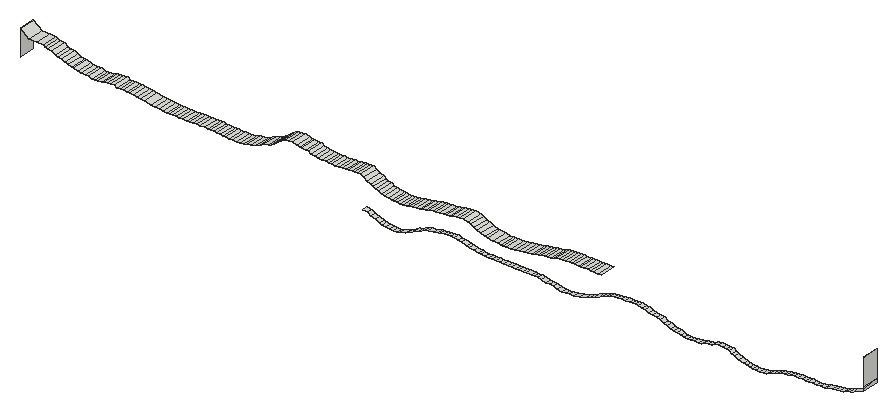
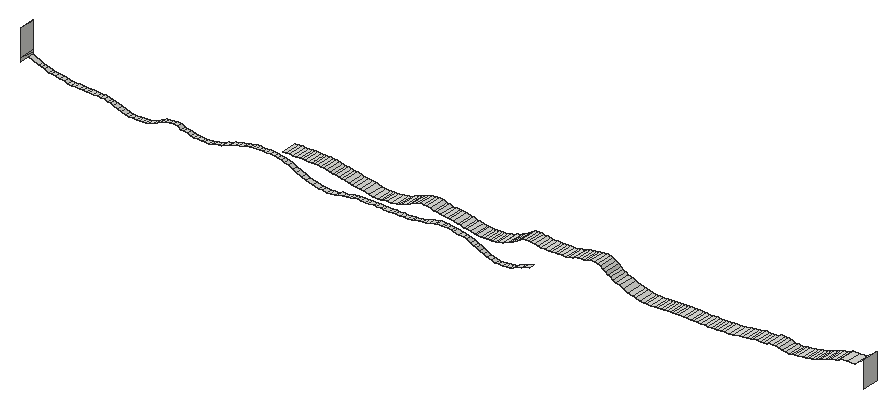
# SketchUp Ruby script. Lengths in inches.
U = 1.inch
M = Sketchup.active_model
def pt(a) = Geom::Point3d.new(a.map { |v| v * U })
def face(e, loops, mat)
  f = e.add_face(loops[0].map { |a| pt(a) })
  loops[1..].each { |l| e.add_face(l.map { |a| pt(a) }).erase! }
  f.material = f.back_material = mat if mat
  f
end
# faces: each face lists its corners as indices into pts; further lists are holes
def faces(e, pts, list, mat = nil) = list.each { |f| face(e, (f[0].is_a?(Array) ? f : [f]).map { |l| l.map { |i| pts[i] } }, mat) }
# xy, xz, yz: faces in a plane at the given z, y or x. An outline is a flat list of corners, or four numbers for a rectangle; further outlines are holes
def ring(l) = l.size == 4 ? [[l[0], l[1]], [l[2], l[1]], [l[2], l[3]], [l[0], l[3]]] : l.each_slice(2).to_a
def flat(e, list, mat, &to3) = list.each { |f| face(e, (f[0].is_a?(Array) ? f : [f]).map { |l| ring(l).map { |u, v| to3.(u, v) } }, mat) }
def xy(e, z, list, mat = nil) = flat(e, list, mat) { |x, y| [x, y, z] }
def xz(e, y, list, mat = nil) = flat(e, list, mat) { |x, z| [x, y, z] }
def yz(e, x, list, mat = nil) = flat(e, list, mat) { |y, z| [x, y, z] }
def lines(e, pts, list) = list.each { |a, b| e.add_line(pt(pts[a]), pt(pts[b])) }
# prism: a flat outline (further loops are holes) pulled along v
def prism(e, loops, v, mat = nil)
  f = face(e, loops, mat); d = Geom::Vector3d.new(v.map { |x| x * U })
  f.pushpull(f.normal.samedirection?(d) ? d.length : -d.length)
end
def box(e, o, s, mat = nil) = prism(e, [[o, [o[0] + s[0], o[1], o[2]], [o[0] + s[0], o[1] + s[1], o[2]], [o[0], o[1] + s[1], o[2]]]], [0, 0, s[2]], mat)
def at(x, y, z, deg = 0) = Geom::Transformation.translation(pt([x, y, z])) * Geom::Transformation.rotation(ORIGIN, Z_AXIS, deg.degrees)
def axes(o, x, y, z) = Geom::Transformation.new([*x, 0, *y, 0, *z, 0, *pt(o).to_a, 1])
def part(name) = M.definitions.add(name)
# library, detail: a bought-in or finely detailed component or shape, given as its bounding box
def library(name, o, s) = part(name).tap { |d| box(d.entities, o, s) }
def detail(e, o, s) = box(e.add_group.entities, o, s)
def put(e, d, t, mat = nil) = e.add_instance(d, t).tap { |i| i.material = mat if mat }
def group(e, t, mat = nil) = e.add_group.tap { |g| g.transformation = t; g.material = mat if mat }.entities
root = M.entities
xy(root,238.18,[[2133.53,2401.37,2134.21,2402.3]])
xy(root,238.62,[[2100.06,2401.37,2100.83,2402.3],[2100.83,2401.37,2101.46,2402.3],[2101.46,2401.37,2102.22,2402.3],[2102.22,2401.37,2102.84,2402.3],[2102.84,2401.37,2103.69,2402.3],
  [2103.69,2401.37,2104.33,2402.3],[2104.33,2401.37,2104.95,2402.3]])
xy(root,238.625,[[2098.64,2401.37,2099.5,2402.3]])
xy(root,238.89,[[2154.45,2401.37,2155.13,2402.3]])
xy(root,238.9,[[2155.89,2401.37,2156.51,2402.3],[2156.51,2401.37,2157.28,2402.3]])
xy(root,240.43,[[2122.73,2401.37,2123.3,2402.3]])
xy(root,241.68,[[2040.78,2401.37,2041.37,2404.3]])
xy(root,241.75,[[2043.13,2401.37,2044,2404.3],[2044,2401.37,2044.62,2404.3],[2044.62,2401.37,2045.13,2404.3]])
xy(root,243.05,[[2115.79,2401.37,2116.47,2404.3]])
xy(root,243.07,[[2113.9375,2401.37,2114.52,2404.3]])
xy(root,243.09,[[2110.625,2401.37,2111.15,2404.3],[2111.15,2401.37,2111.67,2404.3],[2111.67,2401.37,2112.33,2404.3],[2112.33,2401.37,2112.78,2404.3]])
yz(root,2010.34,[[2401.37,241.52,2404.3,246.2]])
yz(root,2164.35,[[2401.37,240.89,2401.37,241.29,2404.3,241.52,2404.3,240.89],[2401.37,241.29,2404.3,241.52,2401.37,241.52],[2401.37,241.52,2401.37,246.27,2402.0625,246.36,2404.3,246.43,2404.3,241.52],[2401.37,246.27,2401.37,246.43,2404.3,246.43,2402.0625,246.36]])
p = [[2077.14,2401.37,237.11],[2077.14,2402.3,237.11],[2077.9,2402.3,237.04],[2077.9,2401.37,237.04],[2078.59,2402.3,237.01],[2078.59,2401.37,237.01],
  [2079.2,2402.3,236.98],[2079.2,2401.37,236.98],[2079.88,2402.3,237.22],[2079.88,2401.37,237.22],[2076.45,2401.37,237.2],[2076.45,2402.3,237.2],
  [2075.92,2401.37,237.33],[2075.92,2402.3,237.33],[2080.73,2402.3,237.43],[2080.73,2401.37,237.43],[2075.25,2401.37,237.68],[2075.25,2402.3,237.68],
  [2081.35,2402.3,237.74],[2081.35,2401.37,237.74],[2144.18,2401.37,237.45],[2144.18,2402.3,237.45],[2144.75,2402.3,237.42],[2144.75,2401.37,237.42],
  [2145.48,2402.3,237.4],[2145.48,2401.37,237.4],[2146.16,2402.3,237.47],[2146.16,2401.37,237.47],[2142.99,2401.37,237.59],[2142.99,2402.3,237.59],
  [2143.59,2402.3,237.51],[2143.59,2401.37,237.51],[2146.76,2402.3,237.5625],[2146.76,2401.37,237.5625],[2142.45,2401.37,237.71],[2142.45,2402.3,237.71],
  [2147.45,2402.3,237.84],[2147.45,2401.37,237.84],[2074.3125,2401.37,237.96],[2074.3125,2402.3,237.96],[2082.05,2402.3,238.02],[2082.05,2401.37,238.02],
  [2109.19,2401.37,237.79],[2109.19,2402.3,237.79],[2109.9,2402.3,237.74],[2109.9,2401.37,237.74],[2110.77,2402.3,237.87],[2110.77,2401.37,237.87],
  [2141.62,2401.37,238],[2141.62,2402.3,238],[2108.42,2401.37,237.86],[2108.42,2402.3,237.86],[2148.13,2402.3,238.08],[2148.13,2401.37,238.08],
  [2107.79,2401.37,238.15],[2107.79,2402.3,238.15],[2111.42,2402.3,237.88],[2111.42,2401.37,237.88],[2112.54,2402.3,238.14],[2112.54,2401.37,238.14],
  [2073.75,2401.37,238.28],[2073.75,2402.3,238.28],[2082.49,2402.3,238.375],[2082.49,2401.37,238.375],[2140.91,2401.37,238.33],[2140.91,2402.3,238.33],
  [2107.02,2401.37,238.19],[2107.02,2402.3,238.19],[2113.76,2402.3,238.46],[2113.76,2401.37,238.46],[2131.51,2401.37,238.19],[2131.51,2402.3,238.19],
  [2132.33,2402.3,238.15],[2132.33,2401.37,238.15],[2132.86,2402.3,238.11],[2132.86,2401.37,238.11],[2133.53,2402.3,238.18],[2133.53,2401.37,238.18],
  [2148.82,2402.3,238.33],[2148.82,2401.37,238.33],[2106.4,2401.37,238.25],[2106.4,2402.3,238.25],[2130.9375,2401.37,238.26],[2130.9375,2402.3,238.26],
  [2134.21,2401.37,238.18],[2134.21,2402.3,238.18],[2134.89,2402.3,238.27],[2134.89,2401.37,238.27],[2072.97,2401.37,238.43],[2072.97,2402.3,238.43],
  [2105.64,2401.37,238.45],[2105.64,2402.3,238.45],[2130.37,2401.37,238.48],[2130.37,2402.3,238.48],[2135.41,2402.3,238.55],[2135.41,2401.37,238.55],
  [2140.36,2401.37,238.57],[2140.36,2402.3,238.57],[2149.35,2402.3,238.51],[2149.35,2401.37,238.51],[2083.05,2402.3,238.51],[2083.05,2401.37,238.51],
  [2083.6875,2402.3,238.76],[2083.6875,2401.37,238.76],[2104.95,2401.37,238.62],[2104.95,2402.3,238.62],[2114.51,2402.3,238.72],[2114.51,2401.37,238.72],
  [2129.71,2401.37,238.56],[2129.71,2402.3,238.56],[2136.07,2402.3,238.61],[2136.07,2401.37,238.61],[2149.92,2402.3,238.6],[2149.92,2401.37,238.6],
  [2095.88,2401.37,238.66],[2095.88,2402.3,238.66],[2096.55,2402.3,238.65],[2096.55,2401.37,238.65],[2097.33,2402.3,238.64],[2097.33,2401.37,238.64],
  [2097.95,2402.3,238.63],[2097.95,2401.37,238.63],[2098.64,2402.3,238.625],[2098.64,2401.37,238.625],[2099.5,2401.37,238.625],[2099.5,2402.3,238.625],
  [2100.06,2402.3,238.62],[2100.06,2401.37,238.62],[2129.14,2401.37,238.67],[2129.14,2402.3,238.67],[2136.66,2402.3,238.66],[2136.66,2401.37,238.66],
  [2139.86,2401.37,238.86],[2139.86,2402.3,238.86],[2150.58,2402.3,238.74],[2150.58,2401.37,238.74],[2094.04,2401.37,238.78],[2094.04,2402.3,238.78],
  [2094.52,2402.3,238.73],[2094.52,2401.37,238.73],[2095.19,2402.3,238.6875],[2095.19,2401.37,238.6875],[2115.39,2402.3,239.08],[2115.39,2401.37,239.08],
  [2128.62,2401.37,239.01],[2128.62,2402.3,239.01],[2137.23,2402.3,239.04],[2137.23,2401.37,239.04],[2151.16,2402.3,238.8],[2151.16,2401.37,238.8],
  [2084.33,2402.3,239.12],[2084.33,2401.37,239.12],[2093.16,2401.37,238.93],[2093.16,2402.3,238.93],[2151.73,2402.3,238.83],[2151.73,2401.37,238.83],
  [2152.47,2402.3,238.86],[2152.47,2401.37,238.86],[2092.39,2401.37,239.07],[2092.39,2402.3,239.07],[2139.34,2401.37,238.96],[2139.34,2402.3,238.96],
  [2153.23,2402.3,238.875],[2153.23,2401.37,238.875],[2153.77,2402.3,238.88],[2153.77,2401.37,238.88],[2154.45,2402.3,238.89],[2154.45,2401.37,238.89],
  [2155.13,2401.37,238.89],[2155.13,2402.3,238.89],[2155.89,2402.3,238.9],[2155.89,2401.37,238.9],[2157.28,2401.37,238.9],[2157.28,2402.3,238.9],
  [2157.91,2402.3,239.15],[2157.91,2401.37,239.15],[2127.9375,2401.37,239.18],[2127.9375,2402.3,239.18],[2137.97,2402.3,239.125],[2137.97,2401.37,239.125],
  [2138.65,2402.3,239.02],[2138.65,2401.37,239.02],[2084.91,2402.3,239.22],[2084.91,2401.37,239.22],[2091.84,2401.37,239.16],[2091.84,2402.3,239.16],
  [2116.18,2402.3,239.375],[2116.18,2401.37,239.375],[2085.91,2402.3,239.31],[2085.91,2401.37,239.31],[2090.99,2401.37,239.44],[2090.99,2402.3,239.44],
  [2127.3125,2401.37,239.5],[2127.3125,2402.3,239.5],[2158.68,2402.3,239.28],[2158.68,2401.37,239.28],[2086.72,2402.3,239.54],[2086.72,2401.37,239.54],
  [2159.48,2402.3,239.42],[2159.48,2401.37,239.42],[2090.32,2401.37,239.56],[2090.32,2402.3,239.56],[2116.92,2402.3,239.75],[2116.92,2401.37,239.75],
  [2160.2,2402.3,239.49],[2160.2,2401.37,239.49],[2087.21,2402.3,239.6],[2087.21,2401.37,239.6],[2126.55,2401.37,239.65],[2126.55,2402.3,239.65],
  [2160.75,2402.3,239.53],[2160.75,2401.37,239.53],[2161.4375,2402.3,239.81],[2161.4375,2401.37,239.81],[2087.83,2402.3,239.65],[2087.83,2401.37,239.65],
  [2088.42,2402.3,239.69],[2088.42,2401.37,239.69],[2089.71,2401.37,239.72],[2089.71,2402.3,239.72],[2088.98,2402.3,239.7],[2088.98,2401.37,239.7],
  [2117.57,2402.3,239.97],[2117.57,2401.37,239.97],[2125.9375,2401.37,239.8],[2125.9375,2402.3,239.8],[2125.18,2401.37,239.96],[2125.18,2402.3,239.96],
  [2161.96,2402.3,239.96],[2161.96,2401.37,239.96],[2118.19,2402.3,240.17],[2118.19,2401.37,240.17],[2124.53,2401.37,240.23],[2124.53,2402.3,240.23],
  [2162.52,2402.3,240.1],[2162.52,2401.37,240.1],[2164.35,2402.3,240.89],[2164.35,2401.37,240.89],[2118.87,2402.3,240.27],[2118.87,2401.37,240.27],
  [2123.95,2401.37,240.27],[2123.95,2402.3,240.27],[2119.55,2402.3,240.33],[2119.55,2401.37,240.33],[2120.24,2402.3,240.37],[2120.24,2401.37,240.37],
  [2123.3,2401.37,240.43],[2123.3,2402.3,240.43],[2120.93,2402.3,240.4],[2120.93,2401.37,240.4],[2121.625,2402.3,240.41],[2121.625,2401.37,240.41],
  [2122.15,2402.3,240.42],[2122.15,2401.37,240.42],[2122.73,2402.3,240.43],[2122.73,2401.37,240.43],[2046.76,2404.3,241.57],[2047.3,2404.3,241.53],
  [2047.3,2401.37,241.53],[2046.76,2401.37,241.57],[2047.92,2404.3,241.51],[2047.92,2401.37,241.51],[2048.47,2404.3,241.49],[2048.47,2401.37,241.49],
  [2049.17,2404.3,241.48],[2049.17,2401.37,241.48],[2049.83,2404.3,241.47],[2049.83,2401.37,241.47],[2050.4,2404.3,241.46],[2050.4,2401.37,241.46],
  [2051.11,2404.3,241.6],[2051.11,2401.37,241.6],[2097.48,2404.3,241.56],[2098.08,2404.3,241.51],[2098.08,2401.37,241.51],[2097.48,2401.37,241.56],
  [2098.53,2404.3,241.48],[2098.53,2401.37,241.48],[2099.05,2404.3,241.46],[2099.05,2401.37,241.46],[2099.92,2404.3,241.51],[2099.92,2401.37,241.51],
  [2100.64,2404.3,241.59],[2100.64,2401.37,241.59],[2046.15,2404.3,241.66],[2046.15,2401.37,241.66],[2051.84,2404.3,241.85],[2051.84,2401.37,241.85],
  [2095.66,2404.3,241.78],[2096.71,2404.3,241.63],[2096.71,2401.37,241.63],[2095.66,2401.37,241.78],[2101.58,2404.3,241.82],[2101.58,2401.37,241.82],
  [2037.12,2404.3,241.75],[2037.57,2404.3,241.74],[2037.57,2401.37,241.74],[2037.12,2401.37,241.75],[2038.12,2404.3,241.72],[2038.12,2401.37,241.72],
  [2038.75,2404.3,241.71],[2038.75,2401.37,241.71],[2039.38,2404.3,241.7],[2039.38,2401.37,241.7],[2040.11,2404.3,241.69],[2040.11,2401.37,241.69],
  [2040.78,2404.3,241.68],[2040.78,2401.37,241.68],[2041.37,2404.3,241.68],[2041.86,2404.3,241.67],[2041.86,2401.37,241.67],[2041.37,2401.37,241.68],
  [2042.5625,2404.3,241.74],[2042.5625,2401.37,241.74],[2043.13,2404.3,241.75],[2043.13,2401.37,241.75],[2045.13,2404.3,241.75],[2045.62,2404.3,241.67],
  [2045.62,2401.37,241.67],[2045.13,2401.37,241.75],[2034.93,2404.3,241.89],[2035.75,2404.3,241.83],[2035.75,2401.37,241.83],[2034.93,2401.37,241.89],
  [2036.35,2404.3,241.78],[2036.35,2401.37,241.78],[2052.51,2404.3,241.91],[2052.51,2401.37,241.91],[2078.14,2404.3,241.89],[2078.6,2404.3,241.85],
  [2078.6,2401.37,241.85],[2078.14,2401.37,241.89],[2079.12,2404.3,241.8125],[2079.12,2401.37,241.8125],[2079.63,2404.3,241.79],[2079.63,2401.37,241.79],
  [2080.21,2404.3,241.78],[2080.21,2401.37,241.78],[2080.88,2404.3,241.91],[2080.88,2401.37,241.91],[2095.17,2404.3,241.89],[2095.17,2401.37,241.89],
  [2102.36,2404.3,241.87],[2102.36,2401.37,241.87],[2034.16,2404.3,241.96],[2034.16,2401.37,241.96],[2053.41,2404.3,242.1],[2053.41,2401.37,242.1],
  [2077.58,2404.3,241.96],[2077.58,2401.37,241.96],[2081.35,2404.3,241.93],[2081.35,2401.37,241.93],[2082.02,2404.3,242.09],[2082.02,2401.37,242.09],
  [2094.53,2404.3,242.14],[2094.53,2401.37,242.14],[2103.125,2404.3,241.98],[2103.125,2401.37,241.98],[2032.99,2404.3,242.24],[2032.99,2401.37,242.24],
  [2076.9,2404.3,242.11],[2076.9,2401.37,242.11],[2103.74,2404.3,242.02],[2103.74,2401.37,242.02],[2104.39,2404.3,242.19],[2104.39,2401.37,242.19],
  [2054.18,2404.3,242.46],[2054.18,2401.37,242.46],[2076.3,2404.3,242.21],[2076.3,2401.37,242.21],[2082.79,2404.3,242.2],[2082.79,2401.37,242.2],
  [2093.77,2404.3,242.39],[2093.77,2401.37,242.39],[2032.32,2404.3,242.34],[2032.32,2401.37,242.34],[2075.79,2404.3,242.51],[2075.79,2401.37,242.51],
  [2083.29,2404.3,242.24],[2083.29,2401.37,242.24],[2083.9,2404.3,242.42],[2083.9,2401.37,242.42],[2105.09,2404.3,242.38],[2105.09,2401.37,242.38],
  [2031.66,2404.3,242.38],[2031.66,2401.37,242.38],[2031,2404.3,242.48],[2031,2401.37,242.48],[2084.45,2404.3,242.47],[2084.45,2401.37,242.47],
  [2093.15,2404.3,242.65],[2093.15,2401.37,242.65],[2105.58,2404.3,242.4375],[2105.58,2401.37,242.4375],[2106.1,2404.3,242.48],[2106.1,2401.37,242.48],
  [2022.82,2404.3,242.68],[2023.49,2404.3,242.51],[2023.49,2401.37,242.51],[2022.82,2401.37,242.68],[2024.01,2404.3,242.46],[2024.01,2401.37,242.46],
  [2024.55,2404.3,242.58],[2024.55,2401.37,242.58],[2030.36,2404.3,242.57],[2030.36,2401.37,242.57],[2054.88,2404.3,242.78],[2054.88,2401.37,242.78],
  [2075.2,2404.3,242.68],[2075.2,2401.37,242.68],[2085.2,2404.3,242.71],[2085.2,2401.37,242.71],[2106.76,2404.3,242.58],[2106.76,2401.37,242.58],
  [2025.18,2404.3,242.57],[2025.18,2401.37,242.57],[2025.81,2404.3,242.81],[2025.81,2401.37,242.81],[2027.58,2404.3,242.92],[2028.01,2404.3,242.625],
  [2028.01,2401.37,242.625],[2027.58,2401.37,242.92],[2028.62,2404.3,242.65],[2028.62,2401.37,242.65],[2029.17,2404.3,242.62],[2029.17,2401.37,242.62],
  [2029.8,2404.3,242.58],[2029.8,2401.37,242.58],[2092.6,2404.3,242.9375],[2092.6,2401.37,242.9375],[2107.29,2404.3,242.61],[2107.29,2401.37,242.61],
  [2107.875,2404.3,242.77],[2107.875,2401.37,242.77],[2021.47,2404.3,242.78],[2022.28,2404.3,242.73],[2022.28,2401.37,242.73],[2021.47,2401.37,242.78],
  [2074.7,2404.3,242.875],[2074.7,2401.37,242.875],[2085.84,2404.3,242.78],[2085.84,2401.37,242.78],[2020.17,2404.3,243.06],[2020.89,2404.3,242.85],
  [2020.89,2401.37,242.85],[2020.17,2401.37,243.06],[2026.38,2404.3,242.86],[2026.38,2401.37,242.86],[2055.65,2404.3,242.97],[2055.65,2401.37,242.97],
  [2086.32,2404.3,242.82],[2086.32,2401.37,242.82],[2087.01,2404.3,242.85],[2087.01,2401.37,242.85],[2108.33,2404.3,242.95],[2108.33,2401.37,242.95],
  [2026.94,2404.3,242.89],[2026.94,2401.37,242.89],[2074.31,2404.3,243.09],[2074.31,2401.37,243.09],[2087.71,2404.3,242.87],[2087.71,2401.37,242.87],
  [2088.26,2404.3,243.02],[2088.26,2401.37,243.02],[2092.03,2404.3,243.14],[2092.03,2401.37,243.14],[2056.18,2404.3,243.23],[2056.18,2401.37,243.23],
  [2088.88,2404.3,243.05],[2088.88,2401.37,243.05],[2108.89,2404.3,243.01],[2108.89,2401.37,243.01],[2109.4,2404.3,243.05],[2109.4,2401.37,243.05],
  [2109.97,2404.3,243.08],[2109.97,2401.37,243.08],[2019.1,2404.3,243.3],[2019.6875,2404.3,243.14],[2019.6875,2401.37,243.14],[2019.1,2401.37,243.3],
  [2073.7,2404.3,243.43],[2073.7,2401.37,243.43],[2089.43,2404.3,243.29],[2089.43,2401.37,243.29],[2091.26,2404.3,243.42],[2091.26,2401.37,243.42],
  [2110.625,2404.3,243.09],[2110.625,2401.37,243.09],[2112.78,2404.3,243.09],[2113.35,2404.3,243.08],[2113.35,2401.37,243.08],[2112.78,2401.37,243.09],
  [2113.9375,2404.3,243.07],[2113.9375,2401.37,243.07],[2114.52,2404.3,243.07],[2115.18,2404.3,243.0625],[2115.18,2401.37,243.0625],[2114.52,2401.37,243.07],
  [2115.79,2404.3,243.05],[2115.79,2401.37,243.05],[2056.58,2404.3,243.48],[2056.58,2401.37,243.48],[2018.46,2404.3,243.48],[2018.46,2401.37,243.48],
  [2090.11,2404.3,243.35],[2090.11,2401.37,243.35],[2073.16,2404.3,243.8],[2073.16,2401.37,243.8],[2090.66,2404.3,243.39],[2090.66,2401.37,243.39],
  [2017.94,2404.3,243.79],[2017.94,2401.37,243.79],[2057.1,2404.3,243.72],[2057.1,2401.37,243.72],[2057.4375,2404.3,244.12],[2057.4375,2401.37,244.12],
  [2017.28,2404.3,243.95],[2017.28,2401.37,243.95],[2072.56,2404.3,244.18],[2072.56,2401.37,244.18],[2016.76,2404.3,244.11],[2016.76,2401.37,244.11],
  [2065.38,2404.3,243.99],[2066.1,2404.3,243.95],[2066.1,2401.37,243.95],[2065.38,2401.37,243.99],[2066.6,2404.3,243.93],[2066.6,2401.37,243.93],
  [2067.29,2404.3,243.91],[2067.29,2401.37,243.91],[2067.86,2404.3,243.89],[2067.86,2401.37,243.89],[2068.56,2404.3,243.88],[2068.56,2401.37,243.88],
  [2069.21,2404.3,243.94],[2069.21,2401.37,243.94],[2069.85,2404.3,243.95],[2069.85,2401.37,243.95],[2070.41,2404.3,244.1],[2070.41,2401.37,244.1],
  [2064.2,2404.3,244.11],[2064.76,2404.3,244.04],[2064.76,2401.37,244.04],[2064.2,2401.37,244.11],[2016.09,2404.3,244.41],[2016.09,2401.37,244.41],
  [2057.91,2404.3,244.39],[2057.91,2401.37,244.39],[2063.45,2404.3,244.25],[2063.45,2401.37,244.25],[2071.04,2404.3,244.13],[2071.04,2401.37,244.13],
  [2071.52,2404.3,244.15],[2071.52,2401.37,244.15],[2072.04,2404.3,244.17],[2072.04,2401.37,244.17],[2062.99,2404.3,244.51],[2062.99,2401.37,244.51],
  [2015.33,2404.3,244.54],[2015.33,2401.37,244.54],[2058.39,2404.3,244.73],[2058.39,2401.37,244.73],[2014.77,2404.3,244.61],[2014.77,2401.37,244.61],
  [2061.84,2404.3,244.67],[2062.45,2404.3,244.55],[2062.45,2401.37,244.55],[2061.84,2401.37,244.67],[2014.55,2404.3,244.92],[2014.55,2401.37,244.92],
  [2058.875,2404.3,244.87],[2058.875,2401.37,244.87],[2060.79,2404.3,244.81],[2061.36,2404.3,244.7],[2061.36,2401.37,244.7],[2060.79,2401.37,244.81],
  [2060.14,2404.3,245.01],[2060.14,2401.37,245.01],[2011.91,2404.3,244.96],[2013.3,2404.3,244.9375],[2013.3,2401.37,244.9375],[2011.91,2401.37,244.96],
  [2059.46,2404.3,244.95],[2059.46,2401.37,244.95],[2010.34,2404.3,246.2],[2010.34,2401.37,246.2]]
faces(root,p,[[0,1,2,3],[3,2,4,5],[5,4,6,7],[7,6,8,9],[10,11,1,0],[12,13,11,10],[9,8,14,15],[16,17,13,12],
  [15,14,18,19],[20,21,22,23],[23,22,24,25],[25,24,26,27],[28,29,30,31],[31,30,21,20],[27,26,32,33],[34,35,29,28],
  [33,32,36,37],[38,39,17,16],[19,18,40,41],[42,43,44,45],[45,44,46,47],[48,49,35,34],[50,51,43,42],[37,36,52,53],
  [54,55,51,50],[47,46,56,57],[57,56,58,59],[60,61,39,38],[41,40,62,63],[64,65,49,48],[66,67,55,54],[59,58,68,69],
  [70,71,72,73],[73,72,74,75],[75,74,76,77],[53,52,78,79],[80,81,67,66],[82,83,71,70],[84,85,86,87],[88,89,61,60],
  [90,91,81,80],[92,93,83,82],[87,86,94,95],[96,97,65,64],[79,78,98,99],[63,62,100,101],[101,100,102,103],[104,105,91,90],
  [69,68,106,107],[108,109,93,92],[95,94,110,111],[99,98,112,113],[114,115,116,117],[117,116,118,119],[119,118,120,121],[121,120,122,123],
  [124,125,126,127],[128,129,109,108],[111,110,130,131],[132,133,97,96],[113,112,134,135],[136,137,138,139],[139,138,140,141],[141,140,115,114],
  [107,106,142,143],[144,145,129,128],[131,130,146,147],[135,134,148,149],[103,102,150,151],[152,153,137,136],[149,148,154,155],[155,154,156,157],
  [158,159,153,152],[160,161,133,132],[157,156,162,163],[163,162,164,165],[165,164,166,167],[168,169,170,171],[172,173,174,175],[176,177,145,144],
  [147,146,178,179],[179,178,180,181],[181,180,161,160],[151,150,182,183],[184,185,159,158],[143,142,186,187],[183,182,188,189],[190,191,185,184],
  [192,193,177,176],[175,174,194,195],[189,188,196,197],[195,194,198,199],[200,201,191,190],[187,186,202,203],[199,198,204,205],[197,196,206,207],
  [208,209,193,192],[205,204,210,211],[211,210,212,213],[207,206,214,215],[215,214,216,217],[218,219,201,200],[217,216,220,221],[221,220,219,218],
  [203,202,222,223],[224,225,209,208],[226,227,225,224],[213,212,228,229],[223,222,230,231],[232,233,227,226],[229,228,234,235],[235,234,236,237],
  [231,230,238,239],[240,241,233,232],[239,238,242,243],[243,242,244,245],[246,247,241,240],[245,244,248,249],[249,248,250,251],[251,250,252,253],
  [253,252,254,255],[256,257,258,259],[257,260,261,258],[260,262,263,261],[262,264,265,263],[264,266,267,265],[266,268,269,267],[268,270,271,269],
  [272,273,274,275],[273,276,277,274],[276,278,279,277],[278,280,281,279],[280,282,283,281],[284,256,259,285],[270,286,287,271],[288,289,290,291],
  [289,272,275,290],[282,292,293,283],[294,295,296,297],[295,298,299,296],[298,300,301,299],[300,302,303,301],[302,304,305,303],[304,306,307,305],
  [308,309,310,311],[309,312,313,310],[312,314,315,313],[316,317,318,319],[317,284,285,318],[320,321,322,323],[321,324,325,322],[324,294,297,325],
  [286,326,327,287],[328,329,330,331],[329,332,333,330],[332,334,335,333],[334,336,337,335],[336,338,339,337],[340,288,291,341],[292,342,343,293],
  [344,320,323,345],[326,346,347,327],[348,328,331,349],[338,350,351,339],[350,352,353,351],[354,340,341,355],[342,356,357,343],[358,344,345,359],
  [360,348,349,361],[356,362,363,357],[362,364,365,363],[346,366,367,347],[368,360,361,369],[352,370,371,353],[372,354,355,373],[374,358,359,375],
  [376,368,369,377],[370,378,379,371],[378,380,381,379],[364,382,383,365],[384,374,375,385],[386,384,385,387],[380,388,389,381],[390,372,373,391],
  [382,392,393,383],[392,394,395,393],[396,397,398,399],[397,400,401,398],[400,402,403,401],[404,386,387,405],[366,406,407,367],[408,376,377,409],
  [388,410,411,389],[394,412,413,395],[402,414,415,403],[414,416,417,415],[418,419,420,421],[419,422,423,420],[422,424,425,423],[424,426,427,425],
  [426,404,405,427],[428,390,391,429],[412,430,431,413],[430,432,433,431],[434,435,436,437],[435,396,399,436],[438,408,409,439],[410,440,441,411],
  [442,443,444,445],[443,434,437,444],[416,446,447,417],[406,448,449,407],[440,450,451,441],[450,452,453,451],[432,454,455,433],[446,456,457,447],
  [456,418,421,457],[458,438,439,459],[452,460,461,453],[460,462,463,461],[464,428,429,465],[448,466,467,449],[462,468,469,463],[454,470,471,455],
  [470,472,473,471],[472,474,475,473],[476,477,478,479],[477,442,445,478],[480,458,459,481],[468,482,483,469],[484,464,465,485],[474,486,487,475],
  [488,489,490,491],[489,492,493,490],[494,495,496,497],[495,498,499,496],[466,500,501,467],[502,476,479,503],[482,504,505,483],[506,480,481,507],
  [504,508,509,505],[508,484,485,509],[510,502,503,511],[500,512,513,501],[512,514,515,513],[516,510,511,517],[518,506,507,519],[520,516,517,521],
  [522,523,524,525],[523,526,527,524],[526,528,529,527],[528,530,531,529],[530,532,533,531],[532,534,535,533],[534,536,537,535],[536,538,539,537],
  [540,541,542,543],[541,522,525,542],[544,520,521,545],[514,546,547,515],[548,540,543,549],[538,550,551,539],[550,552,553,551],[552,554,555,553],
  [554,518,519,555],[556,548,549,557],[558,544,545,559],[546,560,561,547],[562,558,559,563],[564,565,566,567],[565,556,557,566],[568,562,563,569],
  [560,570,571,561],[572,573,574,575],[573,564,567,574],[576,572,575,577],[578,579,580,581],[579,568,569,580],[570,582,583,571],[582,576,577,583],
  [584,578,581,585]])
